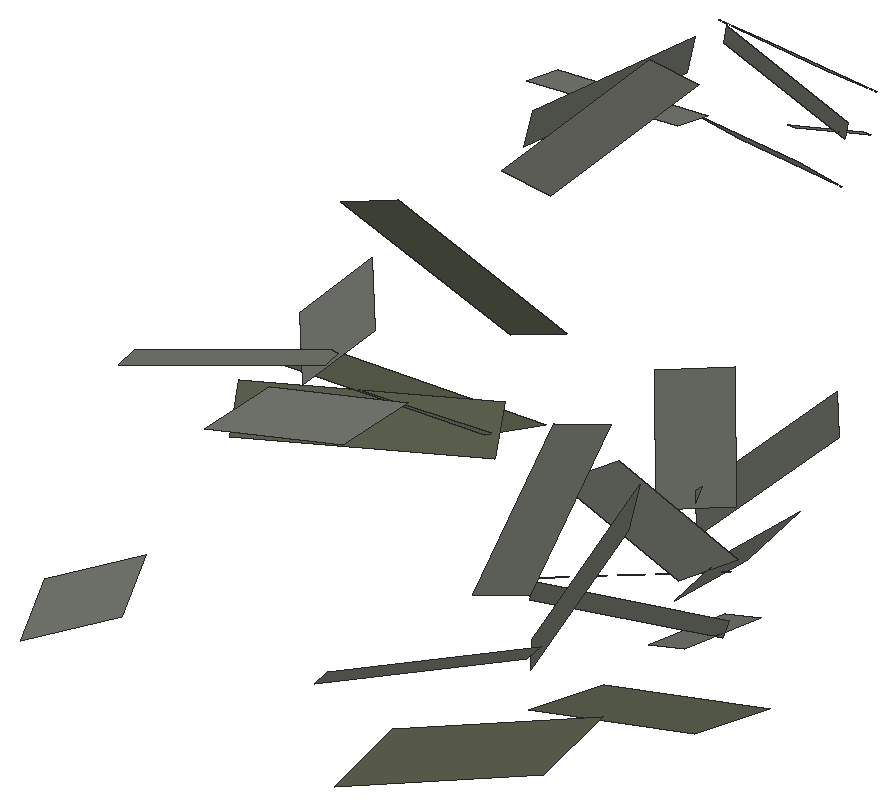
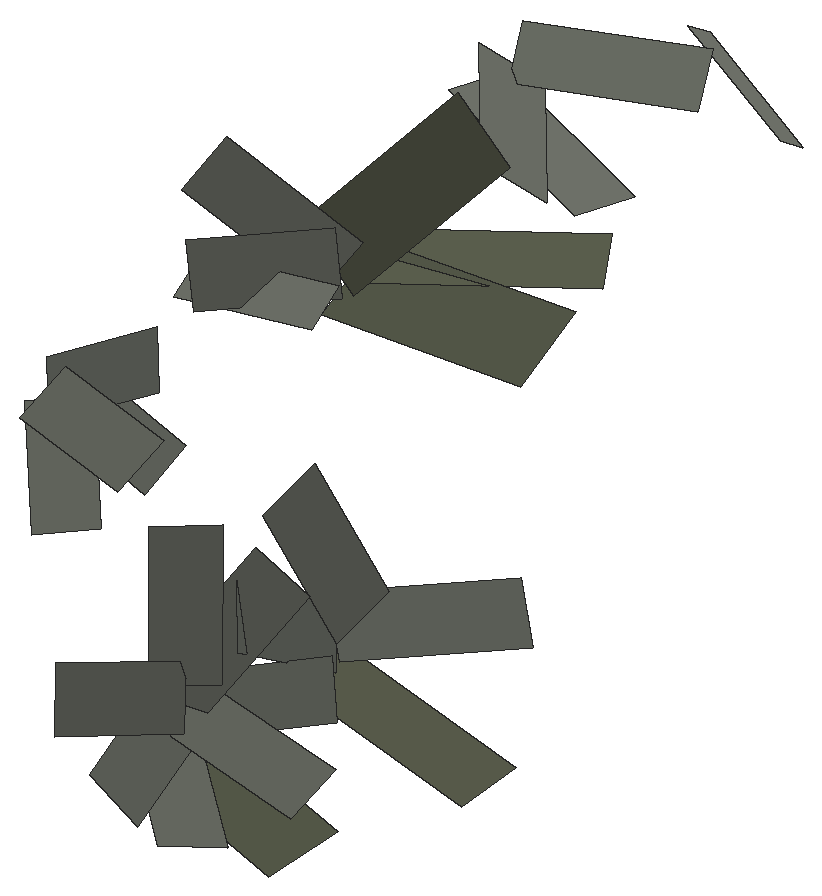
# SketchUp Ruby script. Lengths in inches.
U = 1.inch
M = Sketchup.active_model
def pt(a) = Geom::Point3d.new(a.map { |v| v * U })
def face(e, loops, mat)
  f = e.add_face(loops[0].map { |a| pt(a) })
  loops[1..].each { |l| e.add_face(l.map { |a| pt(a) }).erase! }
  f.material = f.back_material = mat if mat
  f
end
# faces: each face lists its corners as indices into pts; further lists are holes
def faces(e, pts, list, mat = nil) = list.each { |f| face(e, (f[0].is_a?(Array) ? f : [f]).map { |l| l.map { |i| pts[i] } }, mat) }
# xy, xz, yz: faces in a plane at the given z, y or x. An outline is a flat list of corners, or four numbers for a rectangle; further outlines are holes
def ring(l) = l.size == 4 ? [[l[0], l[1]], [l[2], l[1]], [l[2], l[3]], [l[0], l[3]]] : l.each_slice(2).to_a
def flat(e, list, mat, &to3) = list.each { |f| face(e, (f[0].is_a?(Array) ? f : [f]).map { |l| ring(l).map { |u, v| to3.(u, v) } }, mat) }
def xy(e, z, list, mat = nil) = flat(e, list, mat) { |x, y| [x, y, z] }
def xz(e, y, list, mat = nil) = flat(e, list, mat) { |x, z| [x, y, z] }
def yz(e, x, list, mat = nil) = flat(e, list, mat) { |y, z| [x, y, z] }
def lines(e, pts, list) = list.each { |a, b| e.add_line(pt(pts[a]), pt(pts[b])) }
# prism: a flat outline (further loops are holes) pulled along v
def prism(e, loops, v, mat = nil)
  f = face(e, loops, mat); d = Geom::Vector3d.new(v.map { |x| x * U })
  f.pushpull(f.normal.samedirection?(d) ? d.length : -d.length)
end
def box(e, o, s, mat = nil) = prism(e, [[o, [o[0] + s[0], o[1], o[2]], [o[0] + s[0], o[1] + s[1], o[2]], [o[0], o[1] + s[1], o[2]]]], [0, 0, s[2]], mat)
def at(x, y, z, deg = 0) = Geom::Transformation.translation(pt([x, y, z])) * Geom::Transformation.rotation(ORIGIN, Z_AXIS, deg.degrees)
def axes(o, x, y, z) = Geom::Transformation.new([*x, 0, *y, 0, *z, 0, *pt(o).to_a, 1])
def part(name) = M.definitions.add(name)
# library, detail: a bought-in or finely detailed component or shape, given as its bounding box
def library(name, o, s) = part(name).tap { |d| box(d.entities, o, s) }
def detail(e, o, s) = box(e.add_group.entities, o, s)
def put(e, d, t, mat = nil) = e.add_instance(d, t).tap { |i| i.material = mat if mat }
def group(e, t, mat = nil) = e.add_group.tap { |g| g.transformation = t; g.material = mat if mat }.entities
root = M.entities
M.materials.add("viburnumblaasdfas0df1w06d").color = [98, 102, 84]
M.materials.add("viburnumbladsadfasdfad0w122").color = [125, 129, 119]
c1 = part("Component\#315")
p = [[0.25,0,0],[2.05,0.01,0.35],[1.81,4.2,1.66],[0,4.19,1.3125]]
faces(c1.entities,p,[[0,1,2,3]],"viburnumbladsadfasdfad0w122")
c2 = part("viburnumblad2")
put(c2.entities,c1,axes([-19.23,-4.49,-32.18],[83.35428,0,0],[0,79.38502,0],[0,0,83.35428]))
c3 = part("Component\#314")
p = [[0.14,0,0],[2.58,0.05,0.25],[2.44,5.11,2.64],[0,5.05,2.39]]
faces(c3.entities,p,[[0,1,2,3]],"viburnumblaasdfas0df1w06d")
c4 = part("viburnumblad1\#2")
put(c4.entities,c3,axes([-37.25,6.23,19.31],[75.98784,0,0],[0,65.50676,0],[0,0,75.98784]))
put(root,c2,axes([2193.89,268.93,17.95],[-0.00567,0.00572,-0.00867],[-0.00649,-0.01145,-0.00331],[-0.00924,0.00313,0.00728]))
put(root,c2,axes([2194.08,273.83,17.71],[0.00173,0.0098,-0.00563],[-0.00961,-0.00223,-0.00684],[-0.00663,0.00549,0.00752]))
put(root,c2,axes([2194.3,273.49,29.12],[-0.00122,0.00857,-0.00461],[-0.01002,-0.00286,-0.00259],[-0.0035,0.00446,0.00809]))
put(root,c4,axes([2195.67,267.84,15.49],[-0.00086,0.01375,0.00031],[-0.0113,-0.00049,-0.01107],[-0.00962,-0.00074,0.00907]))
put(root,c2,axes([2191.23,272.01,28.18],[0.00614,-0.00518,0.0082],[0.00724,0.00927,0.00063],[-0.0067,0.00499,0.00652]))
put(root,c4,axes([2195.84,265.4,24.87],[-0.00055,0.01258,-0.0057],[-0.01484,-0.00329,-0.00573],[-0.0051,0.00524,0.0099]))
put(root,c2,axes([2194.38,278.76,28.19],[0.00286,0.007,-0.00749],[-0.01015,0.00031,-0.00351],[-0.0019,0.00782,0.00576]))
put(root,c2,axes([2195.05,260.07,29.38],[-0.00445,0.01048,-0.00645],[-0.00976,-0.00718,-0.00494],[-0.00749,0.00313,0.01026]))
put(root,c2,axes([2192.22,270.7,17.875],[0.00076,-0.01192,0.00361],[0.0064,0.00373,0.01004],[-0.01075,0.00137,0.00569]))
put(root,c4,axes([2196.33,265.02,24.84],[-0.00719,0.01195,-0.00129],[-0.01278,-0.0083,-0.00564],[-0.00429,-0.00131,0.01125]))
put(root,c2,axes([2193.95,260.61,28.26],[0.00877,0.00751,0.00615],[-0.00546,0.01067,-0.00523],[-0.00802,0.00094,0.01029]))
put(root,c2,axes([2194.91,252.96,25.875],[-0.00095,0.00927,0.00479],[-0.00714,0.003,-0.00705],[-0.00723,-0.00378,0.00515]))
put(root,c2,axes([2192.82,269.95,16.5625],[0.00644,-0.0055,0.00764],[0.00359,0.01104,0.00474],[-0.00972,-0.00018,0.00726]))
put(root,c4,axes([2195.77,267.65,26.35],[-0.01073,0.0028,-0.00658],[-0.00691,-0.01149,0.00571],[-0.00344,0.00773,0.00806]))
put(root,c2,axes([2195.52,273.67,17.12],[-0.00445,0.00477,-0.00883],[-0.0086,-0.00885,-0.00045],[-0.00678,0.00624,0.00678]))
put(root,c2,axes([2195.15,276.83,27.01],[0.0028,0.00563,-0.00742],[-0.01015,0.00031,-0.00351],[-0.00158,0.00853,0.00492]))
put(root,c2,axes([2194.9,274.79,17.95],[-0.00828,-0.00278,-0.00738],[-0.00265,-0.00909,0.0064],[-0.00743,0.00635,0.00594]))
put(root,c2,axes([2192.46,271.4375,27.63],[-0.00127,-0.00935,0.00568],[0.00996,0.00338,0.00695],[-0.00695,0.00574,0.0058]))
put(root,c2,axes([2193.92,275.95,18.41],[-0.00707,-0.00889,-0.00124],[0.00366,-0.00429,0.00994],[-0.0082,0.00576,0.0055]))
put(root,c2,axes([2195.66,259.87,27.67],[0.00306,0.01272,-0.00021],[-0.01084,0.00248,-0.00806],[-0.00742,0.00196,0.01059]))
put(root,c2,axes([2195.63,277.95,27.67],[-0.00494,0.0045,-0.00826],[-0.00853,-0.00405,0.00272],[-0.002,0.0084,0.00497]))
put(root,c2,axes([2193.48,274.32,16.61],[0.00828,0.00278,0.00738],[0.00071,0.00951,-0.00438],[-0.00785,0.00396,0.00731]))
put(root,c2,axes([2194.23,277.88,27.09],[0.00898,0.00541,-0.00233],[-0.00533,0.00547,-0.00762],[-0.00249,0.00719,0.00626]))
put(root,c2,axes([2194.46,273.44,16.14],[0.00739,0.00929,0.00129],[-0.00498,0.005,-0.00749],[-0.00707,0.00455,0.00775]))
put(root,c2,axes([2192.93,275.8125,17.37],[0.00463,-0.00496,0.0092],[0.00608,0.00946,0.00204],[-0.0085,0.00407,0.00647]))
put(root,c4,axes([2196.62,271.86,14.92],[0.0024,0.01209,-0.00232],[-0.01101,0.00036,-0.0095],[-0.00784,0.00332,0.00921]))
